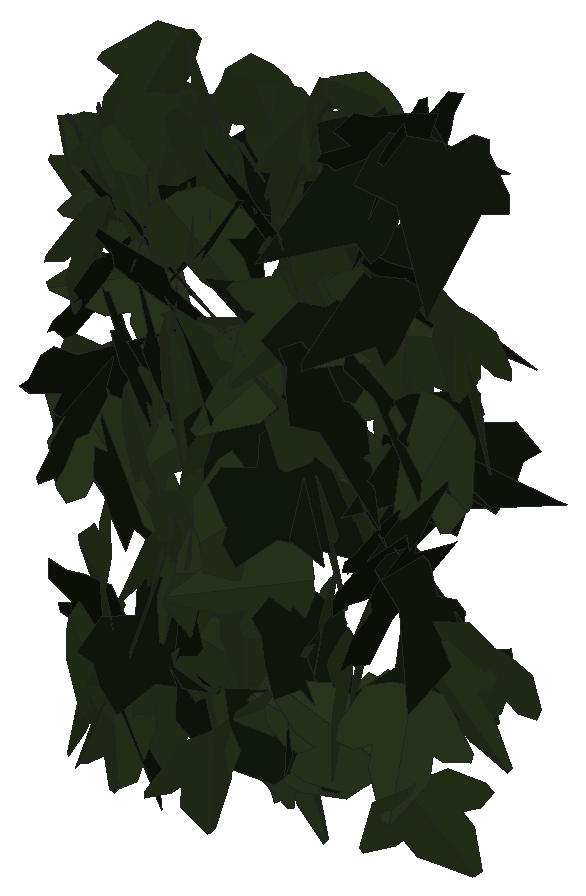
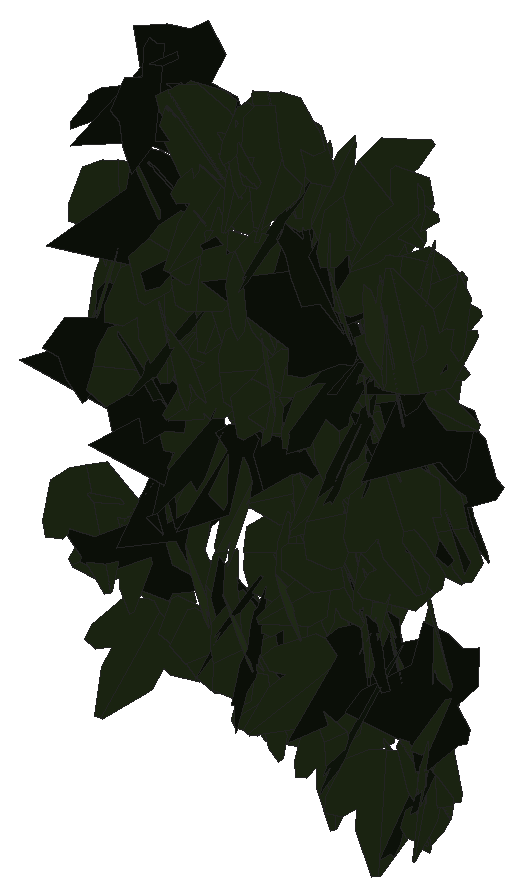
# SketchUp Ruby script. Lengths in inches.
U = 1.inch
M = Sketchup.active_model
def pt(a) = Geom::Point3d.new(a.map { |v| v * U })
def face(e, loops, mat)
  f = e.add_face(loops[0].map { |a| pt(a) })
  loops[1..].each { |l| e.add_face(l.map { |a| pt(a) }).erase! }
  f.material = f.back_material = mat if mat
  f
end
# faces: each face lists its corners as indices into pts; further lists are holes
def faces(e, pts, list, mat = nil) = list.each { |f| face(e, (f[0].is_a?(Array) ? f : [f]).map { |l| l.map { |i| pts[i] } }, mat) }
# xy, xz, yz: faces in a plane at the given z, y or x. An outline is a flat list of corners, or four numbers for a rectangle; further outlines are holes
def ring(l) = l.size == 4 ? [[l[0], l[1]], [l[2], l[1]], [l[2], l[3]], [l[0], l[3]]] : l.each_slice(2).to_a
def flat(e, list, mat, &to3) = list.each { |f| face(e, (f[0].is_a?(Array) ? f : [f]).map { |l| ring(l).map { |u, v| to3.(u, v) } }, mat) }
def xy(e, z, list, mat = nil) = flat(e, list, mat) { |x, y| [x, y, z] }
def xz(e, y, list, mat = nil) = flat(e, list, mat) { |x, z| [x, y, z] }
def yz(e, x, list, mat = nil) = flat(e, list, mat) { |y, z| [x, y, z] }
def lines(e, pts, list) = list.each { |a, b| e.add_line(pt(pts[a]), pt(pts[b])) }
# prism: a flat outline (further loops are holes) pulled along v
def prism(e, loops, v, mat = nil)
  f = face(e, loops, mat); d = Geom::Vector3d.new(v.map { |x| x * U })
  f.pushpull(f.normal.samedirection?(d) ? d.length : -d.length)
end
def box(e, o, s, mat = nil) = prism(e, [[o, [o[0] + s[0], o[1], o[2]], [o[0] + s[0], o[1] + s[1], o[2]], [o[0], o[1] + s[1], o[2]]]], [0, 0, s[2]], mat)
def at(x, y, z, deg = 0) = Geom::Transformation.translation(pt([x, y, z])) * Geom::Transformation.rotation(ORIGIN, Z_AXIS, deg.degrees)
def axes(o, x, y, z) = Geom::Transformation.new([*x, 0, *y, 0, *z, 0, *pt(o).to_a, 1])
def part(name) = M.definitions.add(name)
# library, detail: a bought-in or finely detailed component or shape, given as its bounding box
def library(name, o, s) = part(name).tap { |d| box(d.entities, o, s) }
def detail(e, o, s) = box(e.add_group.entities, o, s)
def put(e, d, t, mat = nil) = e.add_instance(d, t).tap { |i| i.material = mat if mat }
def group(e, t, mat = nil) = e.add_group.tap { |g| g.transformation = t; g.material = mat if mat }.entities
root = M.entities
M.materials.add("efeu1").color = [18, 25, 13]
M.materials.add("efeu2").color = [43, 57, 29]
c1 = part("ivyleaf_10")
p = [[0,0.5,-0.03],[-0.0625,2.02,-0.43],[-0.19,2.01,-0.46],[-0.54,1.05,-0.29],[-0.52,0.625,-0.18],[-0.83,0.76,-0.28],
  [-1.16,0.64,-0.33],[-1.15,0.33,-0.24],[-0.77,-0.39,0.02],[-0.3,-0.51,0.16],[0.04,-0.48,0.23],[-0.02,2.01,-0.4375],
  [-0.06,2.01,-0.43],[0.04,-0.49,0.23],[0.67,-0.49,0.14],[1.38,0.36,-0.2],[1.375,0.51,-0.24],[0.81,0.65,-0.19],
  [0.62,0.59,-0.15],[0.6,1.09,-0.28],[0.5,1.23,-0.31]]
faces(c1.entities,p,[[0,1,2,3,4,5,6,7,8,9,10],[11,12,0,13,14,15,16,17,18,19,20]],"efeu2")
c2 = part("ivyleaf_9")
p = [[1.54,2.16,1.25],[1.36,2.04,1.19],[-0.21,0.99,0.68],[-0.71,1.11,0.82],[-0.85,0.86,0.67],[-0.8,0.17,0.21],
  [-0.9,-0.01,0.1],[-0.67,-0.16,-0.02],[-0.08,-0.08,-0.05],[-0.03,-0.6,-0.4],[0.65,-0.88,-0.66],[0.83,-0.6,-0.49],
  [1.29,-0.42,-0.43],[1.8125,-0.07,-0.26],[1.21,0.44,0.15]]
faces(c2.entities,p,[[0,1,2,3,4,5,6,7,8,9,10,11,12,13,14]],"efeu1")
put(root,c1,axes([22.6,224.3125,212.43],[0.04972,-0.49408,0.05839],[0.01346,-0.05733,-0.49652],[0.49734,0.05094,0.00761]))
put(root,c2,axes([25.72,224.34,213.89],[-0.49356,0.04613,0.06536],[-0.06521,0.00461,-0.49571],[-0.04634,-0.49785,0.00146]))
put(root,c2,axes([25.1,224.32,211.72],[0.23403,-0.43915,-0.04879],[-0.02256,0.04326,-0.49761],[0.44127,0.23511,0.00044]))
put(root,c1,axes([23.25,224.22,209.04],[0.2519,-0.4118,-0.13025],[-0.06978,0.11,-0.48273],[0.42624,0.26138,-0.00205]))
put(root,c1,axes([24.46,224.55,209.29],[-0.02646,-0.00072,0.4993],[-0.25501,-0.42985,-0.01414],[0.42927,-0.2554,0.02238]))
put(root,c1,axes([26.03,224.3,208.61],[0.47948,0.14089,-0.01573],[-0.01625,-0.00051,-0.49974],[-0.14083,0.47974,0.00409]))
put(root,c2,axes([22.62,223.9375,210.39],[-0.08337,0.31997,0.37506],[-0.12373,0.35463,-0.33004],[-0.47722,-0.14784,0.02005]))
put(root,c2,axes([25.95,224.35,212.91],[-0.47351,0.16049,-0.00587],[0.00555,-0.00189,-0.49997],[-0.1605,-0.47354,0.00001]))
put(root,c1,axes([23.13,224.17,210.7],[-0.17494,0.46455,0.05991],[-0.02193,0.05576,-0.4964],[-0.46788,-0.17631,0.00087]))
put(root,c1,axes([25.16,224.57,208.64],[0.14734,-0.26704,0.39621],[0.28263,-0.28559,-0.29758],[0.38524,0.31165,0.06679]))
put(root,c1,axes([24.74,224.52,212.17],[-0.19897,-0.32582,0.32289],[-0.16672,-0.27652,-0.38176],[0.42734,-0.25958,0.0014]))
put(root,c2,axes([24.21,224.16,213.38],[0.44774,-0.01927,-0.22171],[-0.22012,0.03497,-0.44758],[0.03275,0.4984,0.02284]))
put(root,c2,axes([22.95,224.13,211.43],[0.333,-0.07668,-0.36501],[-0.34086,0.13608,-0.33955],[0.15142,0.47498,0.03835]))
put(root,c1,axes([23.3,224.5,209.45],[0.39327,-0.25488,0.17428],[0.14377,-0.0986,-0.46862],[0.27325,0.41871,-0.00427]))
put(root,c1,axes([22.8,224.13,208.9],[-0.02222,0.04405,0.49756],[-0.4472,0.22013,-0.03946],[-0.22253,-0.44677,0.02961]))
put(root,c1,axes([24.78,224.51,213.96],[0.07316,-0.48032,0.11805],[0.01461,-0.11719,-0.48585],[0.4944,0.07454,-0.00311]))
put(root,c1,axes([23.8,224.37,207.47],[-0.1146,-0.48332,-0.05719],[0.02057,0.05389,-0.49666],[0.48626,-0.11619,0.00753]))
put(root,c1,axes([26.37,224.4,211.5],[0.45233,-0.13207,-0.16719],[-0.15817,0.05473,-0.47115],[0.14276,0.47913,0.00774]))
put(root,c2,axes([24.9,224.28,207.79],[-0.39671,-0.01967,0.30371],[0.30365,-0.05935,0.39278],[0.0206,0.49608,0.05903]))
put(root,c1,axes([23.52,224.36,212.68],[-0.38499,-0.02393,-0.31813],[0.31903,-0.03244,-0.38363],[-0.00228,-0.49837,0.04025]))
put(root,c2,axes([22.83,224.33,212.04],[0.44594,-0.13589,0.18076],[0.17759,-0.03698,-0.46593],[0.14,0.47976,0.01528]))
put(root,c1,axes([25.25,224.54,207.84],[0.16346,0.23269,0.41126],[-0.29689,-0.28797,0.28094],[0.36761,-0.33604,0.04403]))
put(root,c1,axes([25.39,224.51,207.95],[0.19209,0.26484,0.37811],[-0.29412,-0.24544,0.32133],[0.35581,-0.34586,0.0615]))
put(root,c2,axes([22.77,224.25,210.08],[0.33999,-0.20354,-0.30492],[-0.24741,0.17951,-0.39568],[0.27055,0.41994,0.02135]))
put(root,c1,axes([23.07,224.64,214.1],[-0.0529,-0.41537,0.27326],[-0.0088,-0.27398,-0.41816],[0.49712,-0.04905,0.02167]))
put(root,c1,axes([24.15,224.04,209.95],[0.05974,0.05905,-0.49289],[0.20995,0.44686,0.07898],[0.44984,-0.2164,0.0286]))
put(root,c1,axes([22.47,224.36,210.16],[0.32616,0.13013,0.35593],[0.33036,0.13248,-0.35116],[-0.18569,0.46424,0.00044]))
put(root,c1,axes([24.7,224.26,213.1],[-0.27859,0.38659,0.15144],[-0.09321,0.11948,-0.47648],[-0.4046,-0.29372,0.0055]))
put(root,c2,axes([25.24,224.51,211.87],[-0.12819,0.01855,0.48293],[-0.47198,0.10266,-0.12923],[-0.10395,-0.489,-0.00881]))
put(root,c1,axes([24.77,224.8,208.2],[-0.01484,-0.00871,-0.4997],[-0.22407,-0.44675,0.01444],[-0.44674,0.22436,0.00936]))
put(root,c2,axes([22.25,224.29,210.54],[0.32063,0.35822,-0.13738],[0.05654,0.13296,0.47867],[0.37947,-0.32248,0.04476]))
put(root,c1,axes([23.28,224.49,211.24],[-0.145,0.45351,-0.15265],[0.04672,-0.14532,-0.47613],[-0.47623,-0.15234,-0.00023]))
put(root,c1,axes([23.74,224.4,213.51],[-0.49618,0.01653,0.05946],[-0.05949,-0.00002,-0.49645],[-0.01641,-0.49973,0.00199]))
put(root,c2,axes([26.23,224.49,211.04],[-0.41776,0.25888,-0.09197],[0.07852,-0.04789,-0.49147],[-0.26327,-0.42507,-0.00064]))
put(root,c1,axes([26.18,224.32,207.76],[-0.32966,-0.29216,-0.23656],[0.1716,0.16299,-0.44044],[0.33448,-0.37158,-0.00719]))
put(root,c2,axes([22.25,224.45,208.33],[0.38265,-0.12843,0.2951],[0.27559,-0.106,-0.4035],[0.16621,0.47145,-0.01033]))
put(root,c1,axes([24.95,224.34,211.21],[-0.3307,-0.09971,-0.36152],[0.34535,0.10693,-0.3454],[0.1462,-0.47815,-0.00185]))
put(root,c2,axes([26.16,224.7,214.1],[-0.11545,-0.4853,-0.03393],[0.00999,0.0325,-0.49884],[0.48639,-0.11586,0.00219]))
put(root,c2,axes([25.93,224.85,209.49],[0.00786,-0.39713,0.30369],[0.02344,-0.3031,-0.39696],[0.49939,0.02048,0.01385]))
put(root,c2,axes([23.12,224.23,208.58],[0.03221,-0.12047,-0.4842],[0.01446,0.48523,-0.11977],[0.49875,-0.00628,0.03475]))
put(root,c1,axes([23.26,224.55,213.58],[-0.28222,-0.40226,0.09243],[-0.05454,-0.07465,-0.49138],[0.40912,-0.28743,-0.00174]))
put(root,c1,axes([26.56,224.42,212.69],[-0.47453,0.03194,0.15428],[-0.15405,0.00862,-0.4756],[-0.03304,-0.4989,0.00166]))
put(root,c1,axes([22.35,224.48,213.04],[-0.41793,0.13077,-0.24132],[0.22714,-0.08202,-0.43781],[-0.15409,-0.47558,0.00915]))
put(root,c1,axes([23.25,224.39,209.45],[0.04175,-0.45198,-0.20969],[-0.01251,0.2094,-0.45387],[0.4981,0.04314,0.00617]))
put(root,c1,axes([24.47,224.43,214.23],[0.45365,-0.10189,-0.18391],[-0.13925,0.18207,-0.44436],[0.15752,0.45439,0.13681]))
put(root,c2,axes([23.1875,224.59,208.54],[-0.14717,0.218,0.42522],[0.17232,-0.39078,0.25999],[0.4457,0.22308,0.03989]))
put(root,c1,axes([22.4,224.33,208.07],[-0.15471,0.44372,0.17083],[-0.05843,0.16054,-0.46991],[-0.47186,-0.16536,0.00218]))
put(root,c1,axes([22.49,224.4,207.09],[0.17801,-0.42498,0.19418],[-0.05932,0.18556,0.46049],[-0.46346,-0.18698,0.01564]))
put(root,c1,axes([23.09,224.52,209.59],[-0.3497,0.32031,-0.15848],[0.11855,-0.1052,-0.47421],[-0.33713,-0.36923,-0.00237]))
put(root,c1,axes([24.43,224.65,207.68],[0.26399,-0.12726,0.40511],[0.40225,-0.07785,-0.28659],[0.13602,0.47723,0.06127]))
put(root,c1,axes([24.12,224.47,208.87],[-0.48318,0.02952,0.12515],[-0.12515,0.00367,-0.48407],[-0.0295,-0.49911,0.00384]))
put(root,c1,axes([22.76,224.41,206.96],[0.3703,-0.1601,0.29538],[-0.27236,0.11435,0.40342],[-0.19673,-0.45966,-0.00252]))
put(root,c1,axes([22.94,224.62,211.82],[0.18603,-0.00001,-0.46411],[-0.46291,-0.03584,-0.18555],[-0.03326,0.49871,-0.01334]))
put(root,c2,axes([23.94,224.53,210.68],[-0.08948,-0.18561,-0.45557],[0.3423,0.30906,-0.19315],[0.3533,-0.34645,0.07176]))
put(root,c1,axes([24.19,224.65,207.67],[0.14689,-0.14704,-0.45476],[0.41718,-0.1927,0.19706],[-0.23321,-0.43732,0.06608]))
put(root,c1,axes([24.3125,224.5,214.09],[-0.48998,-0.07178,-0.06902],[0.0683,0.00996,-0.49521],[0.07247,-0.49472,0.00004]))
put(root,c2,axes([22.51,224.85,207.17],[0.14739,-0.30947,0.36401],[0.14194,-0.33538,-0.3426],[0.45621,0.20433,-0.01101]))
put(root,c1,axes([25.61,224.72,212.46],[0.26404,0.19628,-0.37651],[-0.33771,-0.17166,-0.32632],[-0.25736,0.42662,0.04192]))
put(root,c1,axes([22.96,224.77,211.47],[0.33415,-0.22927,0.29288],[0.23319,-0.17759,-0.40507],[0.28977,0.4073,-0.01176]))
put(root,c1,axes([24.93,224.49,212.45],[-0.4451,-0.18967,-0.12614],[0.11476,0.05243,-0.48382],[0.19676,-0.45965,-0.00314]))
put(root,c1,axes([22.03,224.62,210.48],[0.22334,-0.041,0.44547],[0.4472,0.00758,-0.22351],[0.01157,0.49826,0.04006]))
put(root,c2,axes([24.39,224.35,210.45],[0.02635,-0.13921,-0.47951],[0.10319,0.47133,-0.13116],[0.48853,-0.09205,0.05357]))
put(root,c1,axes([23.83,224.49,213.44],[-0.36795,0.27378,-0.19914],[-0.15912,0.11975,0.45863],[0.29882,0.40088,-0.00099]))
put(root,c2,axes([22.45,224.55,212.43],[0.45222,-0.18656,0.10341],[0.09206,-0.04796,-0.48911],[0.19241,0.46141,-0.00903]))
put(root,c1,axes([25.19,224.375,213.18],[-0.16776,-0.34455,-0.32115],[0.18145,0.26733,-0.38159],[0.43466,-0.24458,0.03534]))
put(root,c1,axes([24.28,224.78,211.39],[0.24896,0.2148,-0.37667],[-0.28061,-0.25131,-0.32878],[-0.33057,0.3751,-0.00458]))
put(root,c1,axes([25.23,224.78,209.07],[0.24944,-0.35232,0.25229],[0.17321,-0.18577,-0.43068],[0.39721,0.30226,0.02937]))
put(root,c1,axes([22.71,224.56,212.47],[-0.34139,0.36276,-0.04312],[-0.0437,0.01805,0.49776],[0.36269,0.34363,0.01938]))
put(root,c1,axes([23.88,224.4,209.3125],[-0.03455,0.01351,0.49862],[-0.47426,0.15398,-0.03703],[-0.15455,-0.47551,0.00218]))
put(root,c2,axes([24.59,224.55,208.96],[0.26158,-0.37113,-0.20938],[-0.10785,0.18002,-0.45383],[0.41224,0.28259,0.01413]))
put(root,c2,axes([25.52,224.28,214.16],[0.38423,0.1812,0.26369],[0.22882,0.13239,-0.4244],[-0.22362,0.44681,0.01881]))
put(root,c1,axes([22.94,224.2,213.53],[-0.02653,0.03577,0.49801],[-0.12654,0.48195,-0.04136],[-0.48299,-0.12823,-0.01652]))
put(root,c2,axes([25.625,224.2,209.98],[-0.0568,0.40493,-0.28776],[-0.0762,0.2791,0.40779],[0.49089,0.09017,0.03001]))
put(root,c1,axes([23.57,224.55,209.57],[-0.21698,-0.41746,0.16926],[0.07493,0.15181,0.47047],[-0.44419,0.22952,-0.00332]))
put(root,c2,axes([26.4,224.83,211.4],[-0.01457,0.08216,-0.49299],[-0.11524,-0.48046,-0.07667],[-0.48632,0.11139,0.03293]))
put(root,c2,axes([25.86,224.8,214.29],[-0.17974,0.22325,-0.4097],[0.25085,-0.32395,-0.28658],[-0.39341,-0.30856,0.00445]))
put(root,c2,axes([23.51,224.87,211.38],[0.43083,-0.23304,-0.10036],[0.08957,-0.04535,0.48982],[-0.2374,-0.44004,0.00267]))
put(root,c1,axes([26.21,224.67,208.91],[-0.30154,0.10963,-0.38348],[0.34594,-0.16736,-0.31987],[-0.19849,-0.45823,0.02509]))
put(root,c1,axes([23.69,224.31,209.24],[-0.07969,-0.1279,-0.47675],[0.28069,0.3855,-0.15034],[0.40603,-0.2916,0.01036]))
put(root,c1,axes([23.95,224.57,211.35],[-0.29087,0.02834,-0.4057],[0.40581,-0.01245,-0.29182],[-0.02665,-0.49904,-0.01576]))
put(root,c1,axes([22.65,224.74,212.41],[-0.38883,-0.07304,-0.30574],[-0.29853,-0.0665,0.39555],[-0.09845,0.49015,0.00811]))
put(root,c2,axes([23.95,224.63,213.03],[-0.33905,0.34573,-0.12458],[0.0814,-0.09465,-0.48417],[-0.35836,-0.34859,0.0079]))
put(root,c1,axes([26.14,224.86,211.01],[0.09819,0.04941,-0.48777],[-0.41859,-0.25052,-0.10964],[-0.25523,0.42988,-0.00783]))
put(root,c2,axes([25.69,224.54,212.69],[0.4338,-0.08365,0.23414],[0.23362,-0.024,-0.44141],[0.08509,0.49237,0.01826]))
put(root,c1,axes([23.23,224.58,212.78],[0.40981,-0.24754,-0.14416],[-0.06282,0.16783,-0.46678],[0.27948,0.4007,0.10645]))
put(root,c1,axes([25.14,224.8,212.24],[-0.46795,0.02839,0.17384],[0.16179,-0.12581,0.45607],[0.06964,0.48308,0.10855]))
put(root,c1,axes([26.74,224.625,209.25],[-0.44477,-0.04124,0.22468],[-0.22349,-0.02317,-0.44667],[0.04725,-0.49776,0.00218]))
put(root,c1,axes([25.76,224.67,211.98],[-0.42937,-0.24869,0.06164],[-0.04992,-0.03678,-0.49614],[0.2513,-0.43221,0.00675]))
put(root,c2,axes([22.46,224.25,211.6],[0.1421,0.32968,0.34802],[0.13223,0.32195,-0.35898],[-0.46079,0.19406,0.00432]))
put(root,c1,axes([23.76,224.29,210.25],[0.01844,0.01606,0.4994],[-0.17477,0.46838,-0.00861],[-0.4681,-0.17425,0.02289]))
put(root,c1,axes([22.8,224.64,213.02],[-0.44424,-0.22849,-0.02116],[0.01846,0.01037,-0.49955],[0.22872,-0.44462,-0.00077]))
put(root,c1,axes([22.41,224.49,207.65],[0.08827,-0.38576,-0.30561],[0.0035,0.31098,-0.39151],[0.49213,0.06698,0.0576]))
put(root,c2,axes([25.36,224.95,211.57],[0.13762,-0.43469,0.2052],[0.09406,-0.18496,-0.45491],[0.47139,0.16381,0.03086]))
put(root,c2,axes([25.72,224.27,209.57],[-0.12604,0.23432,-0.42333],[-0.25749,0.33789,0.26369],[0.40965,0.28448,0.03549]))
put(root,c1,axes([24.74,224.52,214],[-0.00122,-0.41583,-0.27763],[0.04013,0.27666,-0.41455],[0.49839,-0.02329,0.0327]))
put(root,c2,axes([23.16,224.63,210.84],[0.02874,-0.35243,0.35351],[-0.03847,0.35147,0.35353],[-0.49769,-0.04752,-0.00692]))
put(root,c1,axes([24.125,225,211.39],[0.02763,-0.02065,-0.49881],[0.21788,-0.44899,0.03065],[-0.44918,-0.21905,-0.01581]))
put(root,c1,axes([23.3,225.09,210.33],[-0.11745,-0.06965,0.48099],[0.05354,-0.49368,-0.05842],[0.48305,0.03778,0.12342]))
put(root,c1,axes([24.54,224.84,211.52],[-0.10651,0.07036,-0.48343],[-0.47737,-0.1201,0.08769],[-0.10378,0.48024,0.09276]))
put(root,c1,axes([26.4,224.7,212.125],[-0.30259,0.38196,-0.11201],[0.06374,-0.09239,-0.48724],[-0.39291,-0.30915,0.00722]))
put(root,c1,axes([23.82,224.57,207.38],[0.29701,-0.08215,0.39375],[-0.37326,0.12608,0.30786],[-0.14988,-0.47682,0.01357]))
put(root,c1,axes([23.56,224.6875,211.32],[-0.47195,-0.10148,0.13026],[-0.1275,-0.02664,-0.48273],[0.10492,-0.48887,-0.00073]))
put(root,c2,axes([25.1875,224.63,210.58],[0.43381,-0.18644,-0.16446],[-0.15205,0.06271,-0.47217],[0.19669,0.45968,-0.00229]))
put(root,c1,axes([25.23,224.7,210.36],[-0.4579,0.15047,-0.13298],[0.12591,-0.04279,-0.48199],[-0.15643,-0.4749,0.0013]))
put(root,c1,axes([22.87,224.71,212.56],[0.2445,-0.40134,-0.17072],[-0.08782,0.1464,-0.46995],[0.42721,0.25979,0.00109]))
put(root,c2,axes([26.26,224.66,208.56],[-0.49255,-0.08375,0.01947],[0.02055,-0.0047,0.49956],[-0.08349,0.49291,0.00807]))
put(root,c2,axes([23.375,224.875,207.5],[0.08104,-0.45361,0.1941],[-0.02222,0.19314,0.46065],[-0.49289,-0.08329,0.01114]))
put(root,c2,axes([23.0625,225.09,211.09],[0.10944,-0.31448,0.37299],[0.11255,-0.35568,-0.33291],[0.47472,0.15683,-0.00706]))
put(root,c2,axes([25.84,224.6,210.9],[0.178,0.18838,-0.42759],[0.30649,0.2983,0.25901],[0.35268,-0.3543,-0.00928]))
put(root,c2,axes([24.09,224.85,213.3],[0.30466,-0.39349,-0.04841],[-0.02929,0.03855,-0.49765],[0.39538,0.30607,0.00043]))
put(root,c2,axes([24.32,225.08,208.5],[0.00859,0.00194,-0.49992],[0.42732,-0.25953,0.00633],[-0.25947,-0.42736,-0.00612]))
put(root,c1,axes([22.67,224.87,210.7],[-0.32169,-0.35258,0.149],[-0.10262,-0.10807,-0.47727],[0.36876,-0.33765,-0.00284]))
put(root,c1,axes([24.5625,225.02,208.89],[0.27865,-0.28079,0.30579],[0.21527,-0.21718,-0.39559],[0.35499,0.35212,-0.00014]))
put(root,c1,axes([23.29,225,213.05],[0.28181,-0.26387,0.31773],[0.2666,-0.17757,-0.38392],[0.31545,0.3858,0.04062]))
put(root,c1,axes([23.875,225.07,209.46],[0.21204,-0.21425,0.39892],[0.28828,-0.27581,-0.30137],[0.34919,0.35781,0.00657]))
put(root,c1,axes([22.625,225.13,212.55],[0.04615,-0.20677,-0.4529],[0.13263,-0.43329,0.21134],[-0.47987,-0.13964,0.01485]))
put(root,c1,axes([25.35,224.79,214.15],[0.38594,-0.09908,-0.30205],[-0.28551,0.10082,-0.39789],[0.13975,0.4796,0.02124]))
put(root,c1,axes([25.36,224.74,214],[0.19665,0.01642,-0.45941],[-0.44015,0.1509,-0.18302],[0.13264,0.4764,0.07381]))
put(root,c1,axes([22.46,224.78,209.85],[0.32313,-0.01276,-0.38135],[0.38051,-0.02619,0.3233],[-0.02823,-0.49915,-0.00721]))
put(root,c1,axes([25.375,224.95,211.58],[0.41002,-0.2359,0.16196],[0.14151,-0.0788,-0.47304],[0.24871,0.43375,0.00215]))
put(root,c1,axes([24.61,224.86,210.07],[-0.28634,0.35232,-0.20949],[0.13789,-0.15785,-0.45395],[-0.386,-0.31774,-0.00677]))
put(root,c1,axes([22.82,224.8125,207.47],[-0.37599,-0.32919,-0.01611],[0.01218,0.01055,-0.49974],[0.32936,-0.37619,0.00009]))
put(root,c1,axes([22.39,224.86,212.3],[-0.43286,-0.21573,0.12688],[0.11394,0.05582,0.48363],[-0.22283,0.4476,0.00084]))
put(root,c1,axes([24.4,225.01,212.73],[0.07535,-0.46762,0.16017],[0.05594,-0.15291,-0.47275],[0.49111,0.08917,0.02927]))
put(root,c1,axes([23.65,224.67,208.3125],[-0.28585,-0.17982,-0.36872],[0.32259,0.17908,-0.33744],[0.25342,-0.43081,0.01363]))
put(root,c2,axes([23.42,224.74,212.4],[0.22824,-0.02958,0.44388],[0.44264,-0.03475,-0.22992],[0.04445,0.49791,0.01033]))
